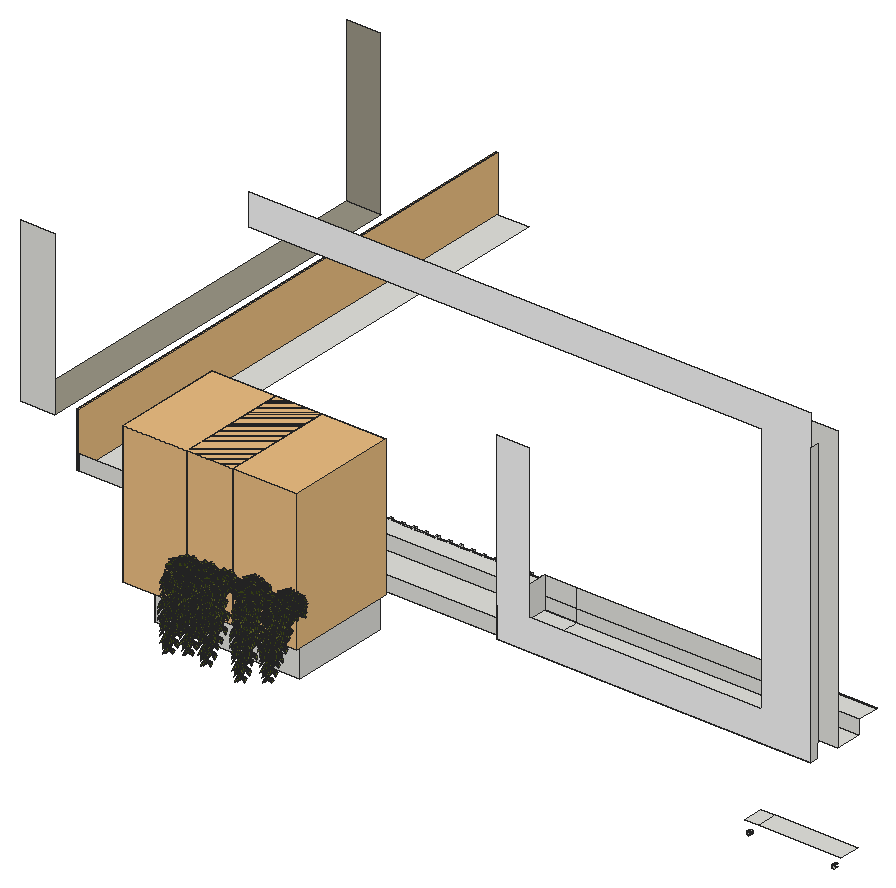
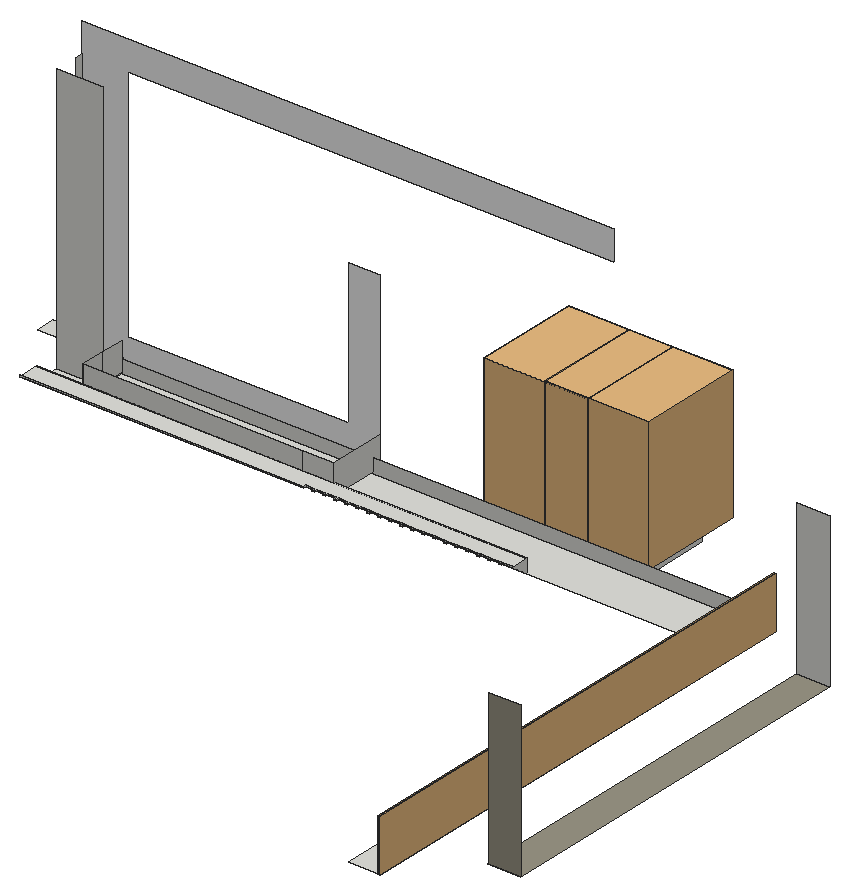
# SketchUp Ruby script. Lengths in inches.
U = 1.inch
M = Sketchup.active_model
def pt(a) = Geom::Point3d.new(a.map { |v| v * U })
def face(e, loops, mat)
  f = e.add_face(loops[0].map { |a| pt(a) })
  loops[1..].each { |l| e.add_face(l.map { |a| pt(a) }).erase! }
  f.material = f.back_material = mat if mat
  f
end
# faces: each face lists its corners as indices into pts; further lists are holes
def faces(e, pts, list, mat = nil) = list.each { |f| face(e, (f[0].is_a?(Array) ? f : [f]).map { |l| l.map { |i| pts[i] } }, mat) }
# xy, xz, yz: faces in a plane at the given z, y or x. An outline is a flat list of corners, or four numbers for a rectangle; further outlines are holes
def ring(l) = l.size == 4 ? [[l[0], l[1]], [l[2], l[1]], [l[2], l[3]], [l[0], l[3]]] : l.each_slice(2).to_a
def flat(e, list, mat, &to3) = list.each { |f| face(e, (f[0].is_a?(Array) ? f : [f]).map { |l| ring(l).map { |u, v| to3.(u, v) } }, mat) }
def xy(e, z, list, mat = nil) = flat(e, list, mat) { |x, y| [x, y, z] }
def xz(e, y, list, mat = nil) = flat(e, list, mat) { |x, z| [x, y, z] }
def yz(e, x, list, mat = nil) = flat(e, list, mat) { |y, z| [x, y, z] }
def lines(e, pts, list) = list.each { |a, b| e.add_line(pt(pts[a]), pt(pts[b])) }
# prism: a flat outline (further loops are holes) pulled along v
def prism(e, loops, v, mat = nil)
  f = face(e, loops, mat); d = Geom::Vector3d.new(v.map { |x| x * U })
  f.pushpull(f.normal.samedirection?(d) ? d.length : -d.length)
end
def box(e, o, s, mat = nil) = prism(e, [[o, [o[0] + s[0], o[1], o[2]], [o[0] + s[0], o[1] + s[1], o[2]], [o[0], o[1] + s[1], o[2]]]], [0, 0, s[2]], mat)
def at(x, y, z, deg = 0) = Geom::Transformation.translation(pt([x, y, z])) * Geom::Transformation.rotation(ORIGIN, Z_AXIS, deg.degrees)
def axes(o, x, y, z) = Geom::Transformation.new([*x, 0, *y, 0, *z, 0, *pt(o).to_a, 1])
def part(name) = M.definitions.add(name)
# library, detail: a bought-in or finely detailed component or shape, given as its bounding box
def library(name, o, s) = part(name).tap { |d| box(d.entities, o, s) }
def detail(e, o, s) = box(e.add_group.entities, o, s)
def put(e, d, t, mat = nil) = e.add_instance(d, t).tap { |i| i.material = mat if mat }
def group(e, t, mat = nil) = e.add_group.tap { |g| g.transformation = t; g.material = mat if mat }.entities
root = M.entities
M.materials.add("[0129_WhiteSmoke]1").color = [245, 245, 245]
M.materials.add("[Concrete Tile]").color = [155, 150, 134]
M.materials.add("asdfasdfasdfasdf").color = [186, 198, 91]
M.materials.add("leaf1_smaller_cleanasdfasfasdfas").color = [88, 95, 33]
M.materials.add("leaf2_smaller_cleansadfasdfasdfasd").color = [55, 66, 19]
c1 = part("glass-railing")
detail(c1.entities,[0,0,0],[1.26,75.59,33.1875])
c2 = library("plant (1)",[-35.72,-28.42,0],[66.31,67.39,84.38])
c3 = part("leaf1a")
p = [[1.06,3.74,11.78],[8.28,8.7,-0.64],[9.51,5.4,26.1],[17.76,4.04,11.26],[17.85,2.23,20],[14.31,3.29,26.73],
  [3.78,3.8125,25.98],[-0.21,2.38,19.72]]
faces(c3.entities,p,[[0,1,2],[2,1,3],[3,4,5],[3,5,2],[6,7,0],[0,2,6]],"leaf1_smaller_cleanasdfasfasdfas")
c4 = part("leaf2a")
p = [[1.4375,3.56,10.81],[8.71,6.8,-0.73],[9.51,3.5,26.59],[16.66,3.91,9.8],[17.86,1.3,19.21],[14.9,1.58,24.92],
  [5.15,2.55,24.01],[1.29,1.87,19.875]]
faces(c4.entities,p,[[0,1,2],[2,1,3],[3,4,5],[3,5,2],[6,7,0],[0,2,6]],"leaf2_smaller_cleansadfasdfasdfasd")
c5 = part("Group\#220")
put(c5.entities,c4,axes([6.68,1.92,2.42],[-0.04671,0.11082,0.08136],[0.07715,0.09226,-0.08136],[-0.11379,0.01705,-0.08856]))
put(c5.entities,c3,axes([1.26,0.54,1.25],[0.13756,-0.04533,0.01029],[0.0079,-0.00888,-0.14471],[0.04581,0.13766,-0.00594]))
put(c5.entities,c4,axes([-0.51,4.89,1.49],[-0.00057,-0.14139,-0.03304],[0.00922,0.03294,-0.14111],[0.14491,-0.00265,0.00885]))
put(c5.entities,c3,axes([4.37,7.98,1.26],[-0.14226,-0.02905,0],[0,0,-0.1452],[0.02905,-0.14226,0]))
put(c5.entities,c3,axes([1.46,4.03,4.07],[0.06242,-0.12847,-0.02614],[-0.10319,-0.03029,-0.09755],[0.08086,0.06051,-0.10432]))
c6 = part("leaf_a")
p = [[1.43,4.41,0.74],[1.39,4.36,0.69],[1.39,4.61,0.21],[1.43,4.67,0.24],[1.35,4.41,0.74],[1.35,4.67,0.24],
  [1.35,3.9,1.02],[1.43,3.9,1.02],[1.39,3.89,0.95],[1.39,3.35,0.9],[1.43,3.34,0.96],[1.35,3.34,0.96]]
faces(c6.entities,p,[[0,1,2,3],[1,4,5,2],[4,0,3,5],[3,2,5],[6,7,0,4],[8,6,4,1],[7,8,1,0],[9,10,11],
  [9,11,6,8],[10,9,8,7],[11,10,7,6]],"asdfasdfasdfasdf")
put(c6.entities,c4,axes([0,-0.08,0.875],[0.1452,0,0],[0,0.02746,-0.14258],[0,0.14258,0.02746]))
c7 = part("leaf_b")
prism(c7.entities,[[[1.36,4.21,-0.25],[1.31,4.13,-0.29],[1.26,4.21,-0.25]]],[0,-0.66,1.14],"asdfasdfasdfasdf")
put(c7.entities,c3,axes([0,-0.1,0.68],[0.1452,-0.0002,0],[0.00006,0.04124,-0.13922],[0.00019,0.13922,0.04124]))
c8 = part("Group\#209")
p = [[2.87,4.13,4.15],[2.98,3.98,4.12],[2.98,4.66,2.59],[2.87,4.8,2.65],[3.09,4.13,4.15],[3.09,4.8,2.65],
  [2.87,4.13,6.07],[2.98,3.98,6.12],[3.09,4.13,6.07],[2.87,5.04,7.34],[2.98,4.91,7.43],[3.09,5.04,7.34]]
faces(c8.entities,p,[[0,1,2,3],[1,4,5,2],[6,7,1,0],[7,8,4,1],[9,10,7,6],[10,11,8,7]],"asdfasdfasdfasdf")
put(c8.entities,c6,axes([0.86,0.51,1.53],[0.95176,-0.27809,0.12967],[0.18405,0.85554,0.48392],[-0.24551,-0.43671,0.86545]))
put(c8.entities,c7,axes([-0.97,2.96,6.52],[0.70711,-0.61237,-0.35355],[0.70711,0.61237,0.35355],[0,-0.5,0.86603]))
put(c8.entities,c6,axes([3.23,0.39,0.41],[0.82736,0.50176,-0.25242],[-0.32519,0.79434,0.5131],[0.45796,-0.34244,0.82037]))
put(c8.entities,c6,axes([3.25,-0.58,4.78],[0.8251,0.44069,-0.35355],[-0.31829,0.8796,0.35355],[0.46679,-0.17918,0.86603]))
c9 = part("Group\#2")
p = [[1.22,4.71,2.14],[1.31,4.57,2.14],[2.16,4.71,3.79],[2.24,4.57,3.77],[1.39,4.71,2.14],[2.33,4.71,3.79],
  [1.93,3.51,6.2],[1.85,3.64,6.23],[2.02,3.64,6.23],[0.93,3.38,8.58],[0.85,3.52,8.58],[1.02,3.52,8.58],
  [0.81,3.57,10.77],[0.72,3.71,10.73],[0.89,3.71,10.73],[1.31,4.57,13.2],[1.22,4.7,13.15],[1.39,4.7,13.15]]
faces(c9.entities,p,[[0,1,2],[3,2,1],[1,4,3],[5,3,4],[6,7,3],[6,3,8],[2,3,7],[5,8,3],
  [9,10,6],[9,6,11],[7,6,10],[8,11,6],[9,11,12],[9,12,10],[13,10,12],[14,12,11],
  [12,15,13],[12,14,15],[16,13,15],[17,15,14]],"asdfasdfasdfasdf")
put(c9.entities,c7,axes([3.93,1.17,1.97],[0.75139,0.49793,0.43299],[-0.65983,0.56085,0.50006],[0.00615,-0.66145,0.74997]))
put(c9.entities,c7,axes([6.23,5.09,1.92],[-0.36585,0.92196,0.12706],[-0.79398,-0.38042,0.47421],[0.48554,0.0726,0.87119]))
put(c9.entities,c7,axes([0.03,0.92,11.26],[1,0,0],[0,0.86603,0.5],[0,-0.5,0.86603]))
put(c9.entities,c6,axes([4.37,2.0625,9.11],[0.45529,0.76896,0.44879],[-0.86129,0.25267,0.44084],[0.22559,-0.58725,0.77733]))
put(c9.entities,c6,axes([1.89,-0.25,4.42],[0.88717,0.14116,0.43931],[-0.36372,0.79981,0.47751],[-0.28396,-0.58342,0.76091]))
put(c9.entities,c6,axes([-0.4,-0.0625,7.9],[0.80178,0.42258,-0.42258],[0,0.70711,0.70711],[0.59763,-0.56694,0.56694]))
put(c9.entities,c7,axes([0.05,0.6875,0.65],[0.97178,0.10445,-0.21151],[0.0126,0.87237,0.48869],[0.23556,-0.47756,0.84643]))
put(c9.entities,c6,axes([5.56,1.19,4.08],[0.24789,0.96746,-0.05068],[-0.86286,0.24427,0.4425],[0.44048,-0.06596,0.89533]))
put(c9.entities,c7,axes([4.91,2.14,7.29],[-0.04249,0.96546,-0.25705],[-0.89911,0.07524,0.4312],[0.43565,0.24944,0.86486]))
c10 = part("Group\#208")
put(c10.entities,c4,axes([5.59,5.52,3.3],[-0.07606,0.12201,-0.02028],[0.09645,0.0436,-0.0994],[-0.07744,-0.06554,-0.10388]))
put(c10.entities,c4,axes([7.69,4.27,1.08],[-0.09839,0.10661,0.00609],[-0.00698,0.00184,-0.14502],[-0.10656,-0.09856,0.00388]))
put(c10.entities,c3,axes([3.51,6.9,2.1],[-0.1403,-0.03711,-0.00465],[-0.00046,0.01976,-0.14385],[0.03739,-0.13898,-0.01921]))
put(c10.entities,c4,axes([2.18,0.07,1.375],[0.14025,0.00096,-0.03757],[-0.03758,0.00358,-0.14021],[0,0.14515,0.00371]))
put(c10.entities,c3,axes([-0.62,2,1.16],[0.081,-0.0806,-0.00996],[0.00004,0.01411,-0.11384],[0.08122,0.08039,0.00999]))
c11 = part("Group\#221")
p = [[1.22,4.71,2.14],[1.31,4.57,2.14],[2.16,4.71,3.79],[2.24,4.57,3.77],[1.39,4.71,2.14],[2.33,4.71,3.79],
  [1.93,3.51,6.2],[1.85,3.64,6.23],[2.02,3.64,6.23],[0.93,3.38,8.58],[0.85,3.52,8.58],[1.02,3.52,8.58],
  [0.81,3.57,10.77],[0.72,3.71,10.73],[0.89,3.71,10.73],[1.31,4.57,13.2],[1.22,4.7,13.15],[1.39,4.7,13.15]]
faces(c11.entities,p,[[0,1,2],[3,2,1],[1,4,3],[5,3,4],[6,7,3],[6,3,8],[2,3,7],[5,8,3],
  [9,10,6],[9,6,11],[7,6,10],[8,11,6],[9,11,12],[9,12,10],[13,10,12],[14,12,11],
  [12,15,13],[12,14,15],[16,13,15],[17,15,14]],"asdfasdfasdfasdf")
put(c11.entities,c7,axes([3.93,1.17,1.97],[0.75139,0.49793,0.43299],[-0.65983,0.56085,0.50006],[0.00615,-0.66145,0.74997]))
put(c11.entities,c7,axes([6.23,5.09,1.92],[-0.36585,0.92196,0.12706],[-0.79398,-0.38042,0.47421],[0.48554,0.0726,0.87119]))
put(c11.entities,c7,axes([0.03,0.92,11.26],[1,0,0],[0,0.86603,0.5],[0,-0.5,0.86603]))
put(c11.entities,c6,axes([4.37,2.0625,9.11],[0.45529,0.76896,0.44879],[-0.86129,0.25267,0.44084],[0.22559,-0.58725,0.77733]))
put(c11.entities,c6,axes([1.89,-0.25,4.42],[0.88717,0.14116,0.43931],[-0.36372,0.79981,0.47751],[-0.28396,-0.58342,0.76091]))
put(c11.entities,c6,axes([-0.4,-0.0625,7.9],[0.80178,0.42258,-0.42258],[0,0.70711,0.70711],[0.59763,-0.56694,0.56694]))
put(c11.entities,c7,axes([0.05,0.6875,0.65],[0.97178,0.10445,-0.21151],[0.0126,0.87237,0.48869],[0.23556,-0.47756,0.84643]))
put(c11.entities,c6,axes([5.56,1.19,4.08],[0.24789,0.96746,-0.05068],[-0.86286,0.24427,0.4425],[0.44048,-0.06596,0.89533]))
put(c11.entities,c7,axes([4.91,2.14,7.29],[-0.04249,0.96546,-0.25705],[-0.89911,0.07524,0.4312],[0.43565,0.24944,0.86486]))
c12 = part("Trailing philodendron")
put(c12.entities,c3,axes([3.65,12.52,19.68],[-0.0527,-0.13492,0.0101],[-0.03487,0.00307,-0.14092],[0.13073,-0.05357,-0.03351]))
put(c12.entities,c3,axes([5.13,11.34,20.6],[-0.03432,-0.12484,0.06572],[-0.08608,-0.03507,-0.11155],[0.11179,-0.06533,-0.06572]))
put(c12.entities,c4,axes([2.61,13.04,18.63],[0.05838,-0.12752,0.03758],[0.01564,-0.03417,-0.14025],[0.13202,0.06044,0]))
put(c12.entities,c4,axes([3.7,9.83,20.73],[-0.00129,-0.14519,0],[-0.0726,0.00064,-0.12575],[0.12574,-0.00112,-0.0726]))
put(c12.entities,c4,axes([11.375,11.11,20.23],[-0.14171,0.00126,0.03163],[-0.02867,0.05638,-0.1307],[-0.01341,-0.1338,-0.05478]))
put(c12.entities,c3,axes([2.4375,12.45,15.12],[-0.02375,-0.14324,0],[0.13106,-0.02173,-0.05859],[0.05781,-0.00958,0.13285]))
put(c12.entities,c3,axes([9.62,10.68,22.01],[0.05693,0.12487,-0.04742],[0.05061,-0.06787,-0.11796],[-0.12361,0.02972,-0.07014]))
put(c12.entities,c3,axes([11.63,16.35,20.5625],[-0.12691,-0.00762,0.07014],[-0.06947,0.03872,-0.12148],[-0.01233,-0.13973,-0.03749]))
put(c12.entities,c3,axes([12.51,17.52,17.81],[-0.1445,0.01001,0.0102],[-0.01383,-0.07182,-0.12544],[-0.0036,-0.1258,0.07242]))
put(c12.entities,c4,axes([9.09,6.34,22.72],[-0.09269,-0.05068,-0.09962],[-0.03661,0.13604,-0.03515],[0.1056,0.00268,-0.09962]))
put(c12.entities,c3,axes([4.83,12.62,22.54],[0.10783,0.09684,-0.00888],[0.09716,-0.10783,0.00397],[-0.00394,-0.00889,-0.14487]))
put(c12.entities,c3,axes([4.94,9.48,20.375],[0.01323,0.07633,0.07653],[0.10803,-0.00667,-0.01203],[-0.00375,0.07738,-0.07653]))
put(c12.entities,c4,axes([14,13.64,21.84],[-0.01852,-0.13907,0.03741],[-0.14373,0.01547,-0.01367],[0.00911,-0.03878,-0.13963]))
put(c12.entities,c4,axes([9.23,4.15,18.71],[0.14198,0.00177,-0.03038],[-0.02867,0.05638,-0.1307],[0.01021,0.13379,0.05548]))
put(c12.entities,c4,axes([5.82,4.5625,15.3],[0.13095,-0.05433,0.03137],[0.06268,0.11013,-0.07089],[0.00273,0.07747,0.12278]))
put(c12.entities,c5,axes([6.59,5.29,16.06],[1.23201,0.26412,0],[-0.26412,1.23201,0],[0,0,1.26]))
put(c12.entities,c8,axes([12.21,1.69,0.66],[-0.82914,0.03045,-0.02227],[0.02366,0.80139,0.21474],[-0.02938,-0.21389,0.80143]))
put(c12.entities,c9,axes([6.8125,1.15,7.57],[0.74375,-0.41052,0.02847],[0.41052,0.73612,-0.11],[0.02847,0.11,0.84237]))
put(c12.entities,c8,axes([-1.68,6.875,13.2],[0.5,-0.86603,0],[0.81585,0.47103,-0.33545],[0.29051,0.16773,0.94206]))
put(c12.entities,c8,axes([1.86,19.56,12.8125],[0.88164,0.4704,0.03781],[0.46333,-0.8476,-0.25863],[0.08962,-0.24554,0.96524]))
g1 = group(c12.entities,at(9.13,11.13,20.67))
put(g1,c4,axes([7.36,4.03,-0.3],[-0.05057,0.11966,-0.06487],[0.07036,-0.03625,-0.12173],[-0.11651,-0.07383,-0.04536]))
put(g1,c4,axes([8.4,1.56,-2.35],[-0.06703,0.12496,-0.03122],[-0.04831,-0.05702,-0.12449],[-0.1194,-0.04708,0.0679]))
put(g1,c3,axes([5.37,5.58,-2.1],[-0.14013,0.0124,0.03596],[-0.03803,-0.04347,-0.13322],[-0.00061,-0.13798,0.0452]))
put(g1,c4,axes([2.45,-0.07,0.8],[0.12002,-0.06072,-0.05468],[-0.07506,-0.04353,-0.11642],[0.03229,0.1245,-0.06737]))
put(g1,c3,axes([0.19,2.38,0.125],[0.05529,-0.09889,0.01797],[-0.03005,-0.03583,-0.10474],[0.09591,0.04578,-0.04318]))
put(c12.entities,c10,axes([17.33,10.54,16.15],[-0.62797,0.46654,0.62289],[-0.59637,-0.80271,0],[0.5,-0.37147,0.78231]))
put(c12.entities,c5,axes([3.44,11.88,17.73],[0.78616,-0.36326,0.5],[0.52263,0.82256,-0.22414],[-0.32986,0.43753,0.83652]))
put(c12.entities,c10,axes([5.5,5.07,16.54],[0.96593,-0.11102,0.2338],[0,0.90334,0.42894],[-0.25882,-0.41432,0.87255]))
put(c12.entities,c8,axes([18.84,3.62,12.91],[-0.80696,-0.59061,0],[-0.57048,0.77946,-0.25882],[-0.15286,0.20886,0.96593]))
put(c12.entities,c9,axes([3.89,0.96,5.21],[0.83948,0.00528,-0.02906],[-0.009,0.83292,-0.10846],[0.02813,0.1087,0.83246]))
put(c12.entities,c9,axes([6.1,0.84,-5.33],[0.875,-0.48296,0.03349],[0.48296,0.86603,-0.12941],[0.03349,0.12941,0.99103]))
put(c12.entities,c9,axes([3.87,-0.55,-8.84],[0.99938,0.00629,-0.0346],[-0.01071,0.99157,-0.12912],[0.03349,0.12941,0.99103]))
put(c12.entities,c8,axes([0.46,6.875,13.01],[0.5,-0.86603,0],[0.81585,0.47103,-0.33545],[0.29051,0.16773,0.94206]))
put(c12.entities,c9,axes([10.39,0.84,1.73],[0.875,-0.48296,0.03349],[0.48296,0.86603,-0.12941],[0.03349,0.12941,0.99103]))
put(c12.entities,c9,axes([-0.75,1.13,2.67],[0.7525,-0.41535,0.0288],[0.41535,0.74478,-0.11129],[0.0288,0.11129,0.85228]))
put(c12.entities,c9,axes([0.04,-0.97,-8.67],[0.735,-0.40569,0.02813],[0.40569,0.72746,-0.1087],[0.02813,0.1087,0.83246]))
put(c12.entities,c9,axes([0.09,-0.6,-7.42],[0.47403,-0.32078,-0.33698],[0.20171,0.57521,-0.26383],[0.41925,0.08595,0.50794]))
put(c12.entities,c9,axes([10.35,0.97,-6.0625],[0.76125,-0.42018,0.02914],[0.42018,0.75344,-0.11259],[0.02914,0.11259,0.86219]))
put(c12.entities,c9,axes([10.78,-1.55,-11.77],[0.72777,-0.42018,0.22517],[0.435,0.75344,0],[-0.19501,0.11259,0.84036]))
put(c12.entities,c9,axes([5.78,-1.55,-20.23],[0.76125,-0.42018,0.02914],[0.42018,0.75344,-0.11259],[0.02914,0.11259,0.86219]))
put(c12.entities,c9,axes([8.72,-1.43,-13.97],[0.65467,-0.36135,0.02506],[0.36135,0.64796,-0.09682],[0.02506,0.09682,0.74149]))
put(c12.entities,c11,axes([1.53,-0.97,-19.86],[0.735,-0.40569,0.02813],[0.40569,0.72746,-0.1087],[0.02813,0.1087,0.83246]))
put(c12.entities,c11,axes([6.23,-2.02,-7.18],[0.55125,-0.30427,0.0211],[0.39555,0.70927,-0.10599],[0.0211,0.08153,0.62435]))
put(c12.entities,c11,axes([6.43,-1.89,6.18],[0.735,-0.40569,0.02813],[0.5274,0.9457,-0.14132],[0.02813,0.1087,0.83246]))
put(c12.entities,c11,axes([10.24,1.09,9.64],[0.62475,-0.34484,0.02391],[0.44829,0.80384,-0.12012],[0.02391,0.0924,0.70759]))
put(c12.entities,c8,axes([1.56,7.74,12.8125],[-0.22619,0.97335,0.03781],[0.93864,0.22817,-0.25863],[0.26037,0.02301,0.96524]))
put(c12.entities,c8,axes([0.65,14.36,12.8125],[0.30411,0.95189,0.03781],[0.92309,-0.28464,-0.25863],[0.23543,-0.11355,0.96524]))
put(c12.entities,c8,axes([7.75,10.38,12.8125],[-0.84074,0.54011,0.03781],[0.51385,0.81797,-0.25863],[0.17062,0.19802,0.96524]))
put(c12.entities,c8,axes([12.92,19.16,12.8125],[0.9234,-0.38197,0.03781],[-0.36017,-0.89632,-0.25863],[-0.13268,-0.22521,0.96524]))
put(c12.entities,c8,axes([6.55,17.22,12.8125],[0.7985,0.60081,0.03781],[0.58857,-0.76596,-0.25863],[0.12643,-0.22877,0.96524]))
put(c12.entities,c8,axes([16.24,8.94,12.8125],[-0.64953,-0.75939,0.03781],[-0.7404,0.62041,-0.25863],[-0.17295,0.19599,0.96524]))
put(c12.entities,c8,axes([15.6875,15.74,12.8125],[0.12972,-0.99083,0.03781],[-0.95648,-0.13509,-0.25863],[-0.26137,0.00261,0.96524]))
put(c12.entities,c8,axes([19.85,8,15.61],[-0.64953,-0.75939,0.03781],[-0.7404,0.62041,-0.25863],[-0.17295,0.19599,0.96524]))
put(c12.entities,c8,axes([18.86,17.5,12.8125],[0.62831,-0.77705,0.03781],[-0.74495,-0.61494,-0.25863],[-0.22422,-0.13434,0.96524]))
put(c12.entities,c8,axes([-0.43,13.28,13.2],[-0.41945,-0.90778,0],[0.85518,-0.39515,-0.33545],[0.30452,-0.14071,0.94206]))
put(c12.entities,c11,axes([4.5625,-2.01,7.45],[0.56595,-0.31238,0.02166],[0.40609,0.72819,-0.10881],[0.02166,0.0837,0.641]))
put(c12.entities,c11,axes([4.48,-2.02,-24.24],[0.55125,-0.30427,0.0211],[0.39555,0.70927,-0.10599],[0.0211,0.08153,0.62435]))
put(c12.entities,c11,axes([4.9,-4.23,-11.04],[0.55125,-0.30427,0.0211],[0.39555,0.70927,-0.10599],[0.0211,0.08153,0.62435]))
put(c12.entities,c10,axes([17.33,10.54,17.41],[-0.62797,0.46654,0.62289],[-0.59637,-0.80271,0],[0.5,-0.37147,0.78231]))
put(c12.entities,c8,axes([-0.03,6.82,20.63],[0.44714,-0.87214,-0.19857],[0.53417,0.43844,-0.7228],[0.71744,0.21712,0.66191]))
put(c12.entities,c8,axes([20.82,12.8,12.8125],[0.12972,-0.99083,0.03781],[-0.95648,-0.13509,-0.25863],[-0.26137,0.00261,0.96524]))
xy(root,138.0625,[[1728.67,801.78,1737.07,814.22],[1737.07,801.78,1786.72,814.22]])
xy(root,138.1875,[[1393.94,776.37,1480.84,836.7]])
xy(root,153.5625,[[1291.04,846.1,1707.86,846.1,1707.86,861.24,1737.07,861.24,1737.07,877.14,1311.45,877.14,1311.45,1160.85,1291.04,1160.85]])
xy(root,154.75,[[1547.79,840.97,1567.4375,877.14],[1567.4375,840.97,1707.86,877.14],[1707.86,840.97,1737.07,845.35]])
xy(root,156.5,[[1232.12,877.14,1252.87,1122.97]],"[Concrete Tile]")
xy(root,162.125,[[1425.1,877.14,1425.1,888.95,1430.52,888.95,1430.52,890.39,1432.16,890.39,1432.16,888.95,1437.58,888.95,1437.58,890.39,1439.16,890.39,1439.16,888.95,1444.58,888.95,1444.58,890.39,1446.16,890.39,1446.16,888.95,1451.58,888.95,1451.58,890.39,1453.16,890.39,1453.16,888.95,1458.58,888.95,1458.58,890.39,1460.16,890.39,1460.16,888.95,1465.58,888.95,1465.58,890.39,1467.16,890.39,1467.16,888.95,1472.58,888.95,1472.58,890.39,1474.16,890.39,1474.16,888.95,1479.58,888.95,1479.58,890.39,1481.16,890.39,1481.16,888.95,1486.58,888.95,1486.58,890.39,1488.16,890.39,1488.16,888.95,1493.58,888.95,1493.58,890.39,1495.16,890.39,1495.16,888.95,1500.58,888.95,1500.58,890.39,1502.16,890.39,1502.16,888.95,1507.58,888.95,1507.58,890.39,1509.16,890.39,1509.16,888.95,1514.58,888.95,1514.58,890.39,1516.16,890.39,1516.16,888.83,1521.58,888.83,1521.58,890.39,1523.16,890.39,1523.16,888.83,1528.58,888.83,1528.58,890.39,1530.16,890.39,1530.16,888.83,1535.58,888.83,1535.58,890.39,1537.16,890.39,1537.16,888.83,1542.58,888.83,1542.58,890.39,1544.16,890.39,1544.16,888.83,1549.58,888.83,1549.58,890.39,1551.16,890.39,1551.16,888.83,1556.58,888.83,1556.58,890.39,1737.07,890.39,1737.07,877.14]])
xz(root,776.37,[[1393.94,138.1875,1480.84,183.3125]])
xz(root,799.91,[[1732.55,131.88,1732.84,131.92,1733.11,132.03,1733.35,132.21,1733.53,132.44,1733.64,132.71,1733.68,133,1733.64,133.29,1733.53,133.57,1733.35,133.8,1733.11,133.98,1732.84,134.09,1732.55,134.13,1732.26,134.09,1731.99,133.98,1731.76,133.8,1731.58,133.57,1731.47,133.29,1731.43,133,1731.47,132.71,1731.58,132.44,1731.76,132.21,1731.99,132.03,1732.26,131.92],[1783.68,131.88,1783.97,131.92,1784.24,132.03,1784.47,132.21,1784.65,132.44,1784.76,132.71,1784.8,133,1784.76,133.29,1784.65,133.57,1784.47,133.8,1784.24,133.98,1783.97,134.09,1783.68,134.13,1783.39,134.09,1783.11,133.98,1782.88,133.8,1782.7,133.57,1782.59,133.29,1782.55,133,1782.59,132.71,1782.7,132.44,1782.88,132.21,1783.11,132.03,1783.39,131.92]])
xz(root,836.7,[[1393.94,138.1875,1480.84,183.3125]])
xz(root,840.97,[[1547.79,154.75,1737.07,154.75,1737.07,343.4375,1398.41,343.4375,1398.41,324.5625,1707.86,324.5625,1707.86,173.4375,1567.4375,173.4375,1567.4375,264.75,1547.79,264.75]],"[0129_WhiteSmoke]1")
xz(root,845.35,[[1707.86,154.75,1737.07,163]])
xz(root,846.1,[[1291.04,153.5625,1707.86,162.75]])
xz(root,861.24,[[1707.86,153.5625,1737.07,324.5625]])
xz(root,877.14,[[1425.1,153.5625,1737.07,153.5625,1737.07,162.125,1707.86,162.125,1707.86,154.75,1547.79,154.75,1547.79,162.125,1425.1,162.125],[1547.79,154.75,1567.4375,162.125],[1567.4375,154.75,1707.86,162.125],[1232.12,156.5,1252.87,254.125],[1547.79,162.125,1567.4375,173.4375],
  [1567.4375,162.125,1707.86,173.4375]])
xz(root,888.83,[[1516.16,162.125,1521.58,162.75],[1523.16,162.125,1528.58,162.75],[1530.16,162.125,1535.58,162.75],[1537.16,162.125,1542.58,162.75],[1544.16,162.125,1549.58,162.75],
  [1551.16,162.125,1556.58,162.75]])
xz(root,888.95,[[1425.1,162.125,1430.52,162.75],[1432.16,162.125,1437.58,162.75],[1439.16,162.125,1444.58,162.75],[1446.16,162.125,1451.58,162.75],[1453.16,162.125,1458.58,162.75],
  [1460.16,162.125,1465.58,162.75],[1467.16,162.125,1472.58,162.75],[1474.16,162.125,1479.58,162.75],[1481.16,162.125,1486.58,162.75],[1488.16,162.125,1493.58,162.75],
  [1495.16,162.125,1500.58,162.75],[1502.16,162.125,1507.58,162.75],[1509.16,162.125,1514.58,162.75]])
xz(root,890.39,[[1430.52,162.125,1432.16,162.75],[1437.58,162.125,1439.16,162.75],[1444.58,162.125,1446.16,162.75],[1451.58,162.125,1453.16,162.75],[1458.58,162.125,1460.16,162.75],
  [1465.58,162.125,1467.16,162.75],[1472.58,162.125,1474.16,162.75],[1479.58,162.125,1481.16,162.75],[1486.58,162.125,1488.16,162.75],[1493.58,162.125,1495.16,162.75],
  [1500.58,162.125,1502.16,162.75],[1507.58,162.125,1509.16,162.75],[1514.58,162.125,1516.16,162.75],[1521.58,162.125,1523.16,162.75],[1528.58,162.125,1530.16,162.75],
  [1535.58,162.125,1537.16,162.75],[1542.58,162.125,1544.16,162.75],[1549.58,162.125,1551.16,162.75],[1556.58,162.125,1559.7,162.75],[1559.7,162.125,1737.07,162.75]])
xz(root,1122.97,[[1232.12,156.5,1252.24,254.125]],"[Concrete Tile]")
yz(root,1393.94,[[776.37,138.1875,836.7,183.3125]])
yz(root,1430.52,[[888.95,162.125,890.39,162.75]])
yz(root,1432.16,[[888.95,162.125,890.39,162.75]])
yz(root,1437.58,[[888.95,162.125,890.39,162.75]])
yz(root,1439.16,[[888.95,162.125,890.39,162.75]])
yz(root,1444.58,[[888.95,162.125,890.39,162.75]])
yz(root,1446.16,[[888.95,162.125,890.39,162.75]])
yz(root,1451.58,[[888.95,162.125,890.39,162.75]])
yz(root,1453.16,[[888.95,162.125,890.39,162.75]])
yz(root,1458.58,[[888.95,162.125,890.39,162.75]])
yz(root,1460.16,[[888.95,162.125,890.39,162.75]])
yz(root,1465.58,[[888.95,162.125,890.39,162.75]])
yz(root,1467.16,[[888.95,162.125,890.39,162.75]])
yz(root,1472.58,[[888.95,162.125,890.39,162.75]])
yz(root,1474.16,[[888.95,162.125,890.39,162.75]])
yz(root,1479.58,[[888.95,162.125,890.39,162.75]])
yz(root,1480.84,[[776.37,138.1875,836.7,183.3125]])
yz(root,1481.16,[[888.95,162.125,890.39,162.75]])
yz(root,1486.58,[[888.95,162.125,890.39,162.75]])
yz(root,1488.16,[[888.95,162.125,890.39,162.75]])
yz(root,1493.58,[[888.95,162.125,890.39,162.75]])
yz(root,1495.16,[[888.95,162.125,890.39,162.75]])
yz(root,1500.58,[[888.95,162.125,890.39,162.75]])
yz(root,1502.16,[[888.95,162.125,890.39,162.75]])
yz(root,1507.58,[[888.95,162.125,890.39,162.75]])
yz(root,1509.16,[[888.95,162.125,890.39,162.75]])
yz(root,1514.58,[[888.95,162.125,890.39,162.75]])
yz(root,1516.16,[[888.83,162.125,890.39,162.75]])
yz(root,1521.58,[[888.83,162.125,890.39,162.75]])
yz(root,1523.16,[[888.83,162.125,890.39,162.75]])
yz(root,1528.58,[[888.83,162.125,890.39,162.75]])
yz(root,1530.16,[[888.83,162.125,890.39,162.75]])
yz(root,1535.58,[[888.83,162.125,890.39,162.75]])
yz(root,1537.16,[[888.83,162.125,890.39,162.75]])
yz(root,1542.58,[[888.83,162.125,890.39,162.75]])
yz(root,1544.16,[[888.83,162.125,890.39,162.75]])
yz(root,1547.79,[[840.97,154.75,877.14,173.4375]])
yz(root,1549.58,[[888.83,162.125,890.39,162.75]])
yz(root,1551.16,[[888.83,162.125,890.39,162.75]])
yz(root,1556.58,[[888.83,162.125,890.39,162.75]])
yz(root,1707.86,[[846.1,153.5625,861.24,154.75],[845.35,154.75,846.1,162.75],[846.1,154.75,861.24,173.4375],[861.24,154.75,877.14,173.4375]])
yz(root,1737.07,[[840.97,154.75,845.35,154.75,845.35,163,846.1,163,846.1,324.5625,840.97,324.5625]])
p = [[1731.99,801.78,132.03],[1732.26,801.78,131.92],[1732.26,799.91,131.92],[1731.99,799.91,132.03],[1732.55,801.78,131.88],[1732.55,799.91,131.88],
  [1732.84,801.78,131.92],[1732.84,799.91,131.92],[1733.11,801.78,132.03],[1733.11,799.91,132.03],[1783.11,801.78,132.03],[1783.39,801.78,131.92],
  [1783.39,799.91,131.92],[1783.11,799.91,132.03],[1783.68,801.78,131.88],[1783.68,799.91,131.88],[1783.97,801.78,131.92],[1783.97,799.91,131.92],
  [1784.24,801.78,132.03],[1784.24,799.91,132.03],[1731.76,801.78,132.21],[1731.76,799.91,132.21],[1733.35,801.78,132.21],[1733.35,799.91,132.21],
  [1782.88,801.78,132.21],[1782.88,799.91,132.21],[1784.47,801.78,132.21],[1784.47,799.91,132.21],[1731.58,801.78,132.44],[1731.58,799.91,132.44],
  [1733.53,801.78,132.44],[1733.53,799.91,132.44],[1782.7,801.78,132.44],[1782.7,799.91,132.44],[1731.47,801.78,132.71],[1731.47,799.91,132.71],
  [1733.64,801.78,132.71],[1733.64,799.91,132.71],[1782.59,801.78,132.71],[1782.59,799.91,132.71],[1731.43,801.78,133],[1731.43,799.91,133],
  [1733.68,801.78,133],[1733.68,799.91,133],[1782.55,801.78,133],[1782.55,799.91,133],[1731.47,801.78,133.29],[1731.47,799.91,133.29],
  [1733.64,801.78,133.29],[1733.64,799.91,133.29],[1782.59,801.78,133.29],[1782.59,799.91,133.29],[1731.58,801.78,133.57],[1731.58,799.91,133.57],
  [1733.53,801.78,133.57],[1733.53,799.91,133.57],[1782.7,801.78,133.57],[1782.7,799.91,133.57],[1731.76,801.78,133.8],[1731.76,799.91,133.8],
  [1733.35,801.78,133.8],[1733.35,799.91,133.8],[1782.88,801.78,133.8],[1782.88,799.91,133.8],[1731.99,801.78,133.98],[1731.99,799.91,133.98],
  [1733.11,801.78,133.98],[1733.11,799.91,133.98],[1783.11,801.78,133.98],[1783.11,799.91,133.98],[1784.47,801.78,133.8],[1784.24,801.78,133.98],
  [1784.24,799.91,133.98],[1784.47,799.91,133.8],[1732.26,801.78,134.09],[1732.26,799.91,134.09],[1732.84,801.78,134.09],[1732.84,799.91,134.09],
  [1783.39,801.78,134.09],[1783.39,799.91,134.09],[1783.97,801.78,134.09],[1783.97,799.91,134.09],[1732.55,801.78,134.13],[1732.55,799.91,134.13],
  [1783.68,801.78,134.13],[1783.68,799.91,134.13]]
faces(root,p,[[0,1,2,3],[1,4,5,2],[4,6,7,5],[6,8,9,7],[10,11,12,13],[11,14,15,12],[14,16,17,15],[16,18,19,17],
  [20,0,3,21],[8,22,23,9],[24,10,13,25],[18,26,27,19],[28,20,21,29],[22,30,31,23],[32,24,25,33],[34,28,29,35],
  [30,36,37,31],[38,32,33,39],[40,34,35,41],[36,42,43,37],[44,38,39,45],[46,40,41,47],[42,48,49,43],[50,44,45,51],
  [52,46,47,53],[48,54,55,49],[56,50,51,57],[58,52,53,59],[54,60,61,55],[62,56,57,63],[64,58,59,65],[60,66,67,61],
  [68,62,63,69],[70,71,72,73],[74,64,65,75],[66,76,77,67],[78,68,69,79],[71,80,81,72],[82,74,75,83],[76,82,83,77],
  [84,78,79,85],[80,84,85,81]])
put(root,c1,axes([1291.04,846.1,153.5625],[1,0,0],[0,4.1738,0],[0,0,1]))
put(root,c2,at(1412.96,800.97,155.86))
put(root,c12,axes([1410.07,757.41,163.27],[1.02772,-0.11891,0],[0.11891,1.02772,0],[0,0,1.03457]))
put(root,c12,axes([1421.29,758.42,164.63],[0.97878,-0.11325,0],[0.11325,0.97878,0],[0,0,0.98531]))
put(root,c12,axes([1432.62,757.84,163.85],[1.00674,-0.11648,0],[0.11648,1.00674,0],[0,0,1.01346]))
put(root,c2,at(1451.52,800.97,155.86))
put(root,c12,axes([1451.74,764.1875,172.43],[0.69913,-0.08089,0],[0.08089,0.69913,0],[0,0,0.70379]))
put(root,c12,axes([1453.32,757.41,163.27],[1.02772,-0.11891,0],[0.11891,1.02772,0],[0,0,1.03457]))
put(root,c12,axes([1468.29,760.14,164.61],[0.94382,-0.1092,0],[0.1092,0.94382,0],[0,0,0.95012]))
put(root,c12,axes([1472.99,764.1875,172.43],[0.69913,-0.08089,0],[0.08089,0.69913,0],[0,0,0.70379]))
